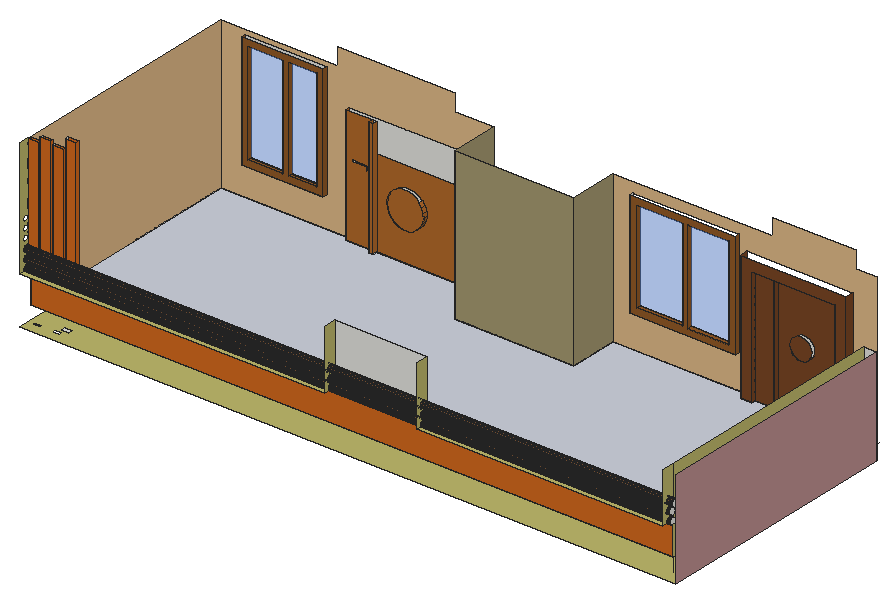
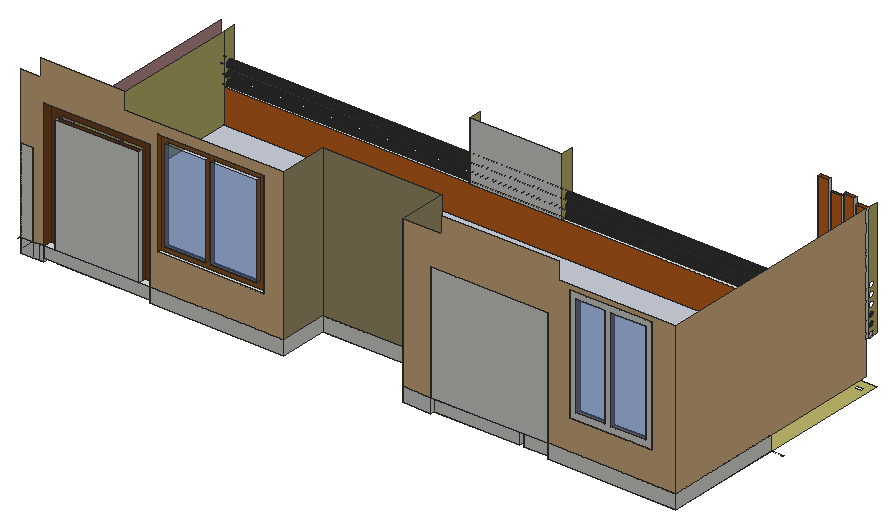
# SketchUp Ruby script. Lengths in inches.
U = 1.inch
M = Sketchup.active_model
def pt(a) = Geom::Point3d.new(a.map { |v| v * U })
def face(e, loops, mat)
  f = e.add_face(loops[0].map { |a| pt(a) })
  loops[1..].each { |l| e.add_face(l.map { |a| pt(a) }).erase! }
  f.material = f.back_material = mat if mat
  f
end
# faces: each face lists its corners as indices into pts; further lists are holes
def faces(e, pts, list, mat = nil) = list.each { |f| face(e, (f[0].is_a?(Array) ? f : [f]).map { |l| l.map { |i| pts[i] } }, mat) }
# xy, xz, yz: faces in a plane at the given z, y or x. An outline is a flat list of corners, or four numbers for a rectangle; further outlines are holes
def ring(l) = l.size == 4 ? [[l[0], l[1]], [l[2], l[1]], [l[2], l[3]], [l[0], l[3]]] : l.each_slice(2).to_a
def flat(e, list, mat, &to3) = list.each { |f| face(e, (f[0].is_a?(Array) ? f : [f]).map { |l| ring(l).map { |u, v| to3.(u, v) } }, mat) }
def xy(e, z, list, mat = nil) = flat(e, list, mat) { |x, y| [x, y, z] }
def xz(e, y, list, mat = nil) = flat(e, list, mat) { |x, z| [x, y, z] }
def yz(e, x, list, mat = nil) = flat(e, list, mat) { |y, z| [x, y, z] }
def lines(e, pts, list) = list.each { |a, b| e.add_line(pt(pts[a]), pt(pts[b])) }
# prism: a flat outline (further loops are holes) pulled along v
def prism(e, loops, v, mat = nil)
  f = face(e, loops, mat); d = Geom::Vector3d.new(v.map { |x| x * U })
  f.pushpull(f.normal.samedirection?(d) ? d.length : -d.length)
end
def box(e, o, s, mat = nil) = prism(e, [[o, [o[0] + s[0], o[1], o[2]], [o[0] + s[0], o[1] + s[1], o[2]], [o[0], o[1] + s[1], o[2]]]], [0, 0, s[2]], mat)
def at(x, y, z, deg = 0) = Geom::Transformation.translation(pt([x, y, z])) * Geom::Transformation.rotation(ORIGIN, Z_AXIS, deg.degrees)
def axes(o, x, y, z) = Geom::Transformation.new([*x, 0, *y, 0, *z, 0, *pt(o).to_a, 1])
def part(name) = M.definitions.add(name)
# library, detail: a bought-in or finely detailed component or shape, given as its bounding box
def library(name, o, s) = part(name).tap { |d| box(d.entities, o, s) }
def detail(e, o, s) = box(e.add_group.entities, o, s)
def put(e, d, t, mat = nil) = e.add_instance(d, t).tap { |i| i.material = mat if mat }
def group(e, t, mat = nil) = e.add_group.tap { |g| g.transformation = t; g.material = mat if mat }.entities
root = M.entities
M.materials.add("[0036_BurlyWood]").color = [222, 184, 135]
M.materials.add("[0041_Chocolate]").color = [210, 105, 30]
M.materials.add("[0057_DarkKhaki]").color = [189, 183, 107]
M.materials.add("[0119_RosyBrown]").color = [188, 143, 143]
M.materials.add("[Marble Carrara Floor Tile]").color = [204, 208, 219]
M.materials.add("[Sandstone]").color = [118, 81, 52]
M.materials.add("[Translucent Glass Blue]").color = [100, 149, 237]
M.materials["[Translucent Glass Blue]"].alpha = 0.5
M.materials.add("[Wood Bamboo]").color = [177, 105, 43]
M.materials.add("[Wood Floor Parquet]").color = [145, 89, 39]
M.materials.add("[Wood Lumber ButtJoined]").color = [164, 152, 112]
M.materials.add("[Wood Veneer 01]").color = [120, 70, 37]
xy(root,229.6875,[[[9,12,9,192.3,100.9,192.3,100.9,189.3,120.23,189.3,120.23,186.3,123.15,186.3,123.15,189.3,184.9,189.3,184.9,192.3,205.37,192.3,205.37,156.87,290.8125,156.87,290.8125,192.3,387.22,192.3,387.22,186.3,395.16,186.3,395.16,189.3,410.94,189.3,410.94,186.3,411.65,186.3,411.65,189.3,455.16,189.3,455.16,186.3,463.09,186.3,463.09,192.3,480,192.3,480,12],[12.36,18.25,17.86,21],[26.86,18.25,32.36,21]]],"[0057_DarkKhaki]")
xy(root,233.5625,[[33.61,18.25,39.11,21]])
xy(root,240,[[120.23,186.3,123.15,189.3],[387.22,186.3,395.16,192.3],[410.94,186.3,411.65,189.3],[455.16,186.3,463.09,192.3],[100.9,189.3,184.9,192.3],
  [395.16,189.3,455.16,192.3]])
xy(root,240,[[9,21,471,21,471,192.3,463.09,192.3,463.09,186.3,455.16,186.3,455.16,189.3,411.65,189.3,411.65,186.3,410.94,186.3,410.94,189.3,395.16,189.3,395.16,186.3,387.22,186.3,387.22,192.3,290.8125,192.3,290.8125,156.87,205.37,156.87,205.37,192.3,184.9,192.3,184.9,189.3,123.15,189.3,123.15,186.3,120.23,186.3,120.23,189.3,100.9,189.3,100.9,192.3,9,192.3]],"[Marble Carrara Floor Tile]")
xy(root,262.28,[[26.03,189.3,84.9,192.3]],"[Wood Floor Parquet]")
xy(root,264,[[9,15.41,227.54,18.4],[227.54,15.41,293.97,18.4],[293.97,15.41,471,18.4],[471,15.41,474.25,18.4],[9,18.4,227.54,18.4,227.54,21,43.6875,21,43.6875,18.8125,35.9375,18.8125,35.9375,21,34.6875,21,34.6875,18.8125,26.9375,18.8125,26.9375,21,25.5,21,25.5,18.8125,17.75,18.8125,17.75,21,16.75,21,16.75,18.8125,9,18.8125],
  [227.54,18.4,293.97,21],[293.97,18.4,471,21],[9,18.8125,16.75,21],[17.75,18.8125,25.5,21]])
xy(root,264,[[9,12,227.54,15.41],[293.97,12,471,15.41]],"[0057_DarkKhaki]")
xy(root,264.7,[[305.18,189.3,381.23,192.3]])
xy(root,266.72,[[30.47,189.3,55.47,192.3],[60.04,189.3,80.47,192.3]],"[Wood Floor Parquet]")
xy(root,269.51,[[309.99,189.3,343.2,192.3],[347.01,189.3,376.42,192.3]],"[Wood Floor Parquet]")
xz(root,18.8125,[[9,264,16.75,348],[17.75,264,25.5,351.875],[26.9375,264,34.6875,349.8125],[35.9375,264,43.6875,357.3125]],"[0041_Chocolate]")
xz(root,21,[[227.54,264,293.97,306.625]])
xz(root,21,[[9,240,9,264,26.9375,264,26.9375,349.8125,34.6875,349.8125,34.6875,264,35.9375,264,35.9375,357.3125,43.6875,357.3125,43.6875,264,471,264,471,240],[9,264,16.75,348],[17.75,264,25.5,351.875]],"[0041_Chocolate]")
xz(root,106.65,[[0,229.6875,9,229.8125]])
xz(root,156.87,[[205.37,229.6875,290.8125,240]])
xz(root,156.87,[[205.37,240,290.8125,348]],"[Wood Lumber ButtJoined]")
xz(root,186.3,[[120.23,229.6875,123.15,240],[387.22,229.6875,395.16,240],[410.94,229.6875,411.65,240],[455.16,229.6875,463.09,240]])
xz(root,186.3,[[120.23,240,123.15,324],[145.13,263.35,148.54,263.51,151.79,264.55,154.66,266.39,156.95,268.91,158.51,271.94,159.24,275.28,159.08,278.68,158.04,281.93,156.19,284.8,153.67,287.09,150.64,288.66,147.31,289.38,143.9,289.22,140.65,288.18,137.79,286.34,135.49,283.8125,133.93,280.78,133.2,277.45,133.37,274.04,134.4,270.8,136.25,267.93,138.77,265.63,141.8,264.07]],"[Wood Bamboo]")
xz(root,186.3,[[387.22,240,395.16,240,395.16,324,455.16,324,455.16,240,463.09,240,463.09,331.9375,387.22,331.9375],[410.94,240,411.65,324],[430.54,279.13,432.55,279.39,434.42,280.17,436.02,281.4,437.26,283,438.03,284.87,438.29,286.88,438.03,288.88,437.26,290.75,436.02,292.36,434.42,293.59,432.55,294.36,430.54,294.63,428.54,294.36,426.67,293.59,425.0625,292.36,423.83,290.75,423.06,288.88,422.79,286.88,423.06,284.87,423.83,283,425.0625,281.4,426.67,280.17,428.54,279.39]],"[Wood Veneer 01]")
xz(root,189.3,[[100.9,229.6875,120.23,240],[123.15,229.6875,184.9,240],[395.16,229.6875,410.94,240],[411.65,229.6875,455.16,240],[120.23,240,123.15,324],
  [410.94,240,411.65,324]])
xz(root,189.3,[[[100.9,240,120.23,324],[115.45,289,115.45,292.0625,105.14,292.0625,105.14,293.5,116.7,293.5,116.7,289]],[[123.15,240,184.9,303.1875],[145.13,263.35,141.8,264.07,138.77,265.63,136.25,267.93,134.4,270.8,133.37,274.04,133.2,277.45,133.93,280.78,135.49,283.8125,137.79,286.34,140.65,288.18,143.9,289.22,147.31,289.38,150.64,288.66,153.67,287.09,156.19,284.8,158.04,281.93,159.08,278.68,159.24,275.28,158.51,271.94,156.95,268.91,154.66,266.39,151.79,264.55,148.54,263.51]]],"[Wood Bamboo]")
xz(root,189.3,[[[26.03,262.28,84.9,344.59],[30.47,266.72,55.47,340.15],[60.04,266.72,80.47,340.15]],[[305.18,264.7,381.23,340.75],[309.99,269.51,343.2,335.94],[347.01,269.51,376.42,335.94]]],"[Wood Floor Parquet]")
xz(root,189.3,[[395.16,240,410.94,324],[[411.65,240,455.16,324],[430.54,279.13,428.54,279.39,426.67,280.17,425.0625,281.4,423.83,283,423.06,284.87,422.79,286.88,423.06,288.88,423.83,290.75,425.0625,292.36,426.67,293.59,428.54,294.36,430.54,294.63,432.55,294.36,434.42,293.59,436.02,292.36,437.26,290.75,438.03,288.88,438.29,286.88,438.03,284.87,437.26,283,436.02,281.4,434.42,280.17,432.55,279.39]]],"[Wood Veneer 01]")
xz(root,192.3,[[9,229.6875,100.9,240],[184.9,229.6875,205.37,240],[290.8125,229.6875,387.22,240],[463.09,229.6875,466.21,240],[466.21,229.6875,471,240],
  [471,229.6875,480,240],[387.22,232.0625,463.09,240],[100.9,240,184.9,324],[395.16,240,455.16,324],[471,240,480,300],
  [[26.03,262.28,84.9,344.59],[30.47,266.72,55.47,340.15],[60.04,266.72,80.47,340.15]]])
xz(root,192.3,[[[9,240,100.9,240,100.9,324,184.9,324,184.9,240,205.37,240,205.37,348,176.74,348,176.74,360,92.74,360,92.74,348,9,348],[26.03,262.28,84.9,344.59]],[[290.8125,240,387.22,240,387.22,331.9375,463.09,331.9375,463.09,240,471,240,471,300,480,300,480,348,465.34,348,465.34,360,405.34,360,405.34,348,290.8125,348],[305.18,264.7,381.23,340.75]]],"[0036_BurlyWood]")
xz(root,192.3,[[30.47,266.72,55.47,340.15],[60.04,266.72,80.47,340.15],[309.99,269.51,343.2,335.94],[347.01,269.51,376.42,335.94]],"[Translucent Glass Blue]")
yz(root,9,[[106.65,229.6875,192.3,240],[16.9,263.4,17.47,263.47,17.99,263.69,18.4,264,15.41,264,15.81,263.69,16.34,263.47],[15.41,264,15.35,264.04,15.01,264.49,14.79,265.02,14.71,265.59,14.79,266.15,15.01,266.68,15.35,267.13,15.81,267.48,16.34,267.7,16.9,267.77,17.47,267.7,17.99,267.48,18.45,267.13,18.8,266.68,18.8125,266.64,18.8125,264.53,18.8,264.49,18.45,264.04,18.4,264],[18.4,264,18.8125,264,18.8125,264.53,18.8,264.49,18.45,264.04],[18.8125,264,18.8125,264.53,19.01,265.02,19.09,265.59,19.01,266.15,18.8125,266.64,18.8125,348,21,348,21,264],
  [18.8125,264.53,18.8125,266.64,19.01,266.15,19.09,265.59,19.01,265.02]])
yz(root,9,[[21,240,192.3,348]],"[0036_BurlyWood]")
yz(root,9,[[[12,264,15.41,264,15.35,264.04,15.01,264.49,14.79,265.02,14.71,265.59,14.79,266.15,15.01,266.68,15.35,267.13,15.81,267.48,16.34,267.7,16.9,267.77,17.47,267.7,17.99,267.48,18.45,267.13,18.8,266.68,18.8125,266.64,18.8125,348,12,348],[16.59,295.27,16.03,295.35,15.5,295.57,15.04,295.91,14.7,296.37,14.48,296.9,14.4,297.46,14.48,298.03,14.7,298.56,15.04,299.01,15.5,299.36,16.03,299.57,16.59,299.65,17.16,299.57,17.69,299.36,18.14,299.01,18.49,298.56,18.7,298.03,18.78,297.46,18.7,296.9,18.49,296.37,18.14,295.91,17.69,295.57,17.16,295.35],[16.59,288.9,16.03,288.97,15.5,289.19,15.04,289.54,14.7,289.99,14.48,290.52,14.4,291.09,14.48,291.65,14.7,292.18,15.04,292.63,15.5,292.98,16.03,293.2,16.59,293.27,17.16,293.2,17.69,292.98,18.14,292.63,18.49,292.18,18.7,291.65,18.78,291.09,18.7,290.52,18.49,289.99,18.14,289.54,17.69,289.19,17.16,288.97],[16.59,282.52,16.03,282.6,15.5,282.82,15.04,283.16,14.7,283.62,14.48,284.15,14.4,284.71,14.48,285.28,14.7,285.81,15.04,286.26,15.5,286.61,16.03,286.82,16.59,286.9,17.16,286.82,17.69,286.61,18.14,286.26,18.49,285.81,18.7,285.28,18.78,284.71,18.7,284.15,18.49,283.62,18.14,283.16,17.69,282.82,17.16,282.6],[16.59,276.15,16.03,276.22,15.5,276.44,15.04,276.79,14.7,277.24,14.48,277.77,14.4,278.34,14.48,278.9,14.7,279.43,15.04,279.88,15.5,280.23,16.03,280.45,16.59,280.52,17.16,280.45,17.69,280.23,18.14,279.88,18.49,279.43,18.7,278.9,18.78,278.34,18.7,277.77,18.49,277.24,18.14,276.79,17.69,276.44,17.16,276.22],[16.59,269.77,16.03,269.85,15.5,270.07,15.04,270.41,14.7,270.87,14.48,271.4,14.4,271.96,14.48,272.53,14.7,273.06,15.04,273.51,15.5,273.86,16.03,274.07,16.59,274.15,17.16,274.07,17.69,273.86,18.14,273.51,18.49,273.06,18.7,272.53,18.78,271.96,18.7,271.4,18.49,270.87,18.14,270.41,17.69,270.07,17.16,269.85]]],"[0057_DarkKhaki]")
yz(root,16.75,[[18.8125,264,21,348]],"[0041_Chocolate]")
yz(root,17.75,[[18.8125,264,21,351.875]])
yz(root,25.5,[[18.8125,264,21,351.875]],"[0041_Chocolate]")
yz(root,26.03,[[189.3,262.28,192.3,344.59]],"[Wood Floor Parquet]")
yz(root,26.9375,[[18.8125,264,21,349.8125]])
yz(root,30.47,[[189.3,266.72,192.3,340.15]],"[Wood Floor Parquet]")
yz(root,34.6875,[[18.8125,264,21,349.8125]],"[0041_Chocolate]")
yz(root,35.9375,[[18.8125,264,21,357.3125]])
yz(root,43.6875,[[18.8125,264,21,357.3125]],"[0041_Chocolate]")
yz(root,55.47,[[189.3,266.72,192.3,340.15]],"[Wood Floor Parquet]")
yz(root,60.04,[[189.3,266.72,192.3,340.15]],"[Wood Floor Parquet]")
yz(root,80.47,[[189.3,266.72,192.3,340.15]],"[Wood Floor Parquet]")
yz(root,84.9,[[189.3,262.28,192.3,344.59]],"[Wood Floor Parquet]")
yz(root,100.9,[[189.3,229.6875,192.3,240]])
yz(root,100.9,[[189.3,240,192.3,324]],"[Wood Bamboo]")
yz(root,120.23,[[186.3,229.6875,189.3,240]])
yz(root,120.23,[[186.3,240,189.3,324]],"[Wood Bamboo]")
yz(root,123.15,[[186.3,229.6875,189.3,240]])
yz(root,123.15,[[186.3,240,189.3,324]],"[Wood Bamboo]")
yz(root,184.9,[[189.3,229.6875,192.3,240]])
yz(root,184.9,[[189.3,240,192.3,324]],"[Wood Bamboo]")
yz(root,205.37,[[156.87,229.6875,192.3,240]])
yz(root,205.37,[[156.87,240,192.3,348]],"[Wood Lumber ButtJoined]")
yz(root,227.54,[[12,264,21,306.625]],"[0057_DarkKhaki]")
yz(root,290.8125,[[156.87,229.6875,192.3,240]])
yz(root,290.8125,[[156.87,240,192.3,348]],"[Wood Lumber ButtJoined]")
yz(root,293.97,[[12,264,21,306.625]],"[0057_DarkKhaki]")
yz(root,305.18,[[189.3,264.7,192.3,340.75]])
yz(root,309.99,[[189.3,269.51,192.3,335.94]],"[Wood Floor Parquet]")
yz(root,343.2,[[189.3,269.51,192.3,335.94]],"[Wood Floor Parquet]")
yz(root,347.01,[[189.3,269.51,192.3,335.94]],"[Wood Floor Parquet]")
yz(root,376.42,[[189.3,269.51,192.3,335.94]],"[Wood Floor Parquet]")
yz(root,381.23,[[189.3,264.7,192.3,340.75]],"[Wood Floor Parquet]")
yz(root,387.22,[[186.3,229.6875,192.3,240]])
yz(root,387.22,[[186.3,240,192.3,331.9375]],"[Wood Veneer 01]")
yz(root,395.16,[[186.3,229.6875,189.3,240],[189.3,240,192.3,324]])
yz(root,395.16,[[186.3,240,189.3,324]],"[Wood Veneer 01]")
yz(root,410.94,[[186.3,229.6875,189.3,240]])
yz(root,410.94,[[186.3,240,189.3,324]],"[Wood Veneer 01]")
yz(root,411.65,[[186.3,229.6875,189.3,240]])
yz(root,411.65,[[186.3,240,189.3,324]],"[Wood Veneer 01]")
yz(root,455.16,[[186.3,229.6875,189.3,240],[189.3,240,192.3,324]])
yz(root,455.16,[[186.3,240,189.3,324]],"[Wood Veneer 01]")
yz(root,463.09,[[186.3,229.6875,192.3,240]])
yz(root,463.09,[[186.3,240,192.3,331.9375]],"[Wood Veneer 01]")
yz(root,471,[[21,240,192.3,300],[12,264,21,300]],"[0057_DarkKhaki]")
yz(root,473.8125,[[16.59,269.77,17.16,269.85,17.69,270.07,18.14,270.41,18.49,270.87,18.7,271.4,18.78,271.96,18.7,272.53,18.49,273.06,18.14,273.51,17.69,273.86,17.16,274.07,16.59,274.15,16.03,274.07,15.5,273.86,15.04,273.51,14.7,273.06,14.48,272.53,14.4,271.96,14.48,271.4,14.7,270.87,15.04,270.41,15.5,270.07,16.03,269.85]])
yz(root,474.25,[[15.41,264,18.4,264,18.45,264.04,18.8,264.49,19.01,265.02,19.09,265.59,19.01,266.15,18.8,266.68,18.45,267.13,17.99,267.48,17.47,267.7,16.9,267.77,16.34,267.7,15.81,267.48,15.35,267.13,15.01,266.68,14.79,266.15,14.71,265.59,14.79,265.02,15.01,264.49,15.35,264.04]])
yz(root,476.125,[[16.59,276.15,17.16,276.22,17.69,276.44,18.14,276.79,18.49,277.24,18.7,277.77,18.78,278.34,18.7,278.9,18.49,279.43,18.14,279.88,17.69,280.23,17.16,280.45,16.59,280.52,16.03,280.45,15.5,280.23,15.04,279.88,14.7,279.43,14.48,278.9,14.4,278.34,14.48,277.77,14.7,277.24,15.04,276.79,15.5,276.44,16.03,276.22]])
yz(root,480,[[12,229.6875,192.3,300]],"[0119_RosyBrown]")
p = [[141.8,189.3,264.07],[145.13,189.3,263.35],[145.13,186.3,263.35],[141.8,186.3,264.07],[148.54,189.3,263.51],[148.54,186.3,263.51],
  [151.79,189.3,264.55],[151.79,186.3,264.55],[9,15.01,264.49],[9,15.35,264.04],[474.25,15.35,264.04],[474.25,15.01,264.49],
  [9,15.41,264],[227.54,15.41,264],[293.97,15.41,264],[471,15.41,264],[474.25,15.41,264],[9,18.4,264],
  [9,18.45,264.04],[474.25,18.45,264.04],[474.25,18.4,264],[471,18.4,264],[293.97,18.4,264],[227.54,18.4,264],
  [9,18.8,264.49],[474.25,18.8,264.49],[138.77,189.3,265.63],[138.77,186.3,265.63],[9,14.79,265.02],[474.25,14.79,265.02],
  [9,18.8125,264.53],[9,19.01,265.02],[474.25,19.01,265.02],[154.66,189.3,266.39],[154.66,186.3,266.39],[9,14.71,265.59],
  [474.25,14.71,265.59],[9,19.09,265.59],[474.25,19.09,265.59],[9,14.79,266.15],[474.25,14.79,266.15],[9,19.01,266.15],
  [474.25,19.01,266.15],[136.25,189.3,267.93],[136.25,186.3,267.93],[9,15.01,266.68],[474.25,15.01,266.68],[9,18.8125,266.64],
  [9,18.8,266.68],[474.25,18.8,266.68],[156.95,189.3,268.91],[156.95,186.3,268.91],[9,15.35,267.13],[474.25,15.35,267.13],
  [9,18.45,267.13],[474.25,18.45,267.13],[9,15.81,267.48],[474.25,15.81,267.48],[9,17.99,267.48],[474.25,17.99,267.48],
  [9,16.34,267.7],[474.25,16.34,267.7],[9,17.47,267.7],[474.25,17.47,267.7],[9,16.9,267.77],[474.25,16.9,267.77],
  [134.4,189.3,270.8],[134.4,186.3,270.8],[158.51,189.3,271.94],[158.51,186.3,271.94],[9,15.5,270.07],[9,16.03,269.85],
  [473.8125,16.03,269.85],[473.8125,15.5,270.07],[9,16.59,269.77],[473.8125,16.59,269.77],[9,17.16,269.85],[473.8125,17.16,269.85],
  [9,17.69,270.07],[473.8125,17.69,270.07],[9,15.04,270.41],[473.8125,15.04,270.41],[9,18.14,270.41],[473.8125,18.14,270.41],
  [9,14.7,270.87],[473.8125,14.7,270.87],[9,18.49,270.87],[473.8125,18.49,270.87],[133.37,189.3,274.04],[133.37,186.3,274.04],
  [9,14.48,271.4],[473.8125,14.48,271.4],[9,18.7,271.4],[473.8125,18.7,271.4],[9,14.4,271.96],[473.8125,14.4,271.96],
  [9,18.78,271.96],[473.8125,18.78,271.96],[159.24,189.3,275.28],[159.24,186.3,275.28],[9,14.48,272.53],[473.8125,14.48,272.53],
  [9,18.7,272.53],[473.8125,18.7,272.53],[9,14.7,273.06],[473.8125,14.7,273.06],[9,18.49,273.06],[473.8125,18.49,273.06],
  [9,15.04,273.51],[473.8125,15.04,273.51],[9,18.14,273.51],[473.8125,18.14,273.51],[9,15.5,273.86],[473.8125,15.5,273.86],
  [9,17.69,273.86],[473.8125,17.69,273.86],[9,16.03,274.07],[473.8125,16.03,274.07],[9,17.16,274.07],[473.8125,17.16,274.07],
  [133.2,189.3,277.45],[133.2,186.3,277.45],[9,16.59,274.15],[473.8125,16.59,274.15],[159.08,189.3,278.68],[159.08,186.3,278.68],
  [9,16.03,276.22],[9,16.59,276.15],[476.125,16.59,276.15],[476.125,16.03,276.22],[9,17.16,276.22],[476.125,17.16,276.22],
  [9,15.5,276.44],[476.125,15.5,276.44],[9,17.69,276.44],[476.125,17.69,276.44],[9,15.04,276.79],[476.125,15.04,276.79],
  [9,18.14,276.79],[476.125,18.14,276.79],[9,14.7,277.24],[476.125,14.7,277.24],[9,18.49,277.24],[476.125,18.49,277.24],
  [9,14.48,277.77],[476.125,14.48,277.77],[9,18.7,277.77],[476.125,18.7,277.77],[133.93,189.3,280.78],[133.93,186.3,280.78],
  [9,14.4,278.34],[476.125,14.4,278.34],[9,18.78,278.34],[476.125,18.78,278.34],[9,14.48,278.9],[476.125,14.48,278.9],
  [9,18.7,278.9],[476.125,18.7,278.9],[158.04,189.3,281.93],[158.04,186.3,281.93],[9,14.7,279.43],[476.125,14.7,279.43],
  [9,18.49,279.43],[476.125,18.49,279.43],[428.54,189.3,279.39],[430.54,189.3,279.13],[430.54,186.3,279.13],[428.54,186.3,279.39],
  [432.55,189.3,279.39],[432.55,186.3,279.39],[9,15.04,279.88],[476.125,15.04,279.88],[9,18.14,279.88],[476.125,18.14,279.88],
  [426.67,189.3,280.17],[426.67,186.3,280.17],[434.42,189.3,280.17],[434.42,186.3,280.17],[9,15.5,280.23],[476.125,15.5,280.23],
  [9,17.69,280.23],[476.125,17.69,280.23],[9,16.03,280.45],[476.125,16.03,280.45],[9,17.16,280.45],[476.125,17.16,280.45],
  [425.0625,189.3,281.4],[425.0625,186.3,281.4],[436.02,189.3,281.4],[436.02,186.3,281.4],[9,16.59,280.52],[476.125,16.59,280.52],
  [135.49,189.3,283.8125],[135.49,186.3,283.8125],[423.83,189.3,283],[423.83,186.3,283],[437.26,189.3,283],[437.26,186.3,283],
  [156.19,189.3,284.8],[156.19,186.3,284.8],[471,316.59,240],[480,316.59,240],[480,195.03,240],[480,192.3,240],
  [471,195.03,240],[471,192.3,240],[471,201.23,240],[471,21,240],[471,21,229.6875]]
faces(root,p,[[0,1,2,3],[1,4,5,2],[4,6,7,5],[26,0,3,27],[6,33,34,7],[43,26,27,44],[33,50,51,34],[66,43,44,67],
  [50,68,69,51],[88,66,67,89],[68,98,99,69],[120,88,89,121],[98,124,125,99],[148,120,121,149],[124,158,159,125],[192,148,149,193],
  [158,198,199,159]],"[Wood Bamboo]")
faces(root,p,[[8,9,10,11],[9,12,13,14,15,16,10],[17,18,19,20,21,22,23],[18,24,25,19],[28,8,11,29],[30,31,32,25,24],[35,28,29,36],[31,37,38,32],
  [39,35,36,40],[37,41,42,38],[45,39,40,46],[47,48,49,42,41],[52,45,46,53],[48,54,55,49],[56,52,53,57],[54,58,59,55],
  [60,56,57,61],[58,62,63,59],[64,60,61,65],[62,64,65,63],[70,71,72,73],[71,74,75,72],[74,76,77,75],[76,78,79,77],
  [80,70,73,81],[78,82,83,79],[84,80,81,85],[82,86,87,83],[90,84,85,91],[86,92,93,87],[94,90,91,95],[92,96,97,93],
  [100,94,95,101],[96,102,103,97],[104,100,101,105],[102,106,107,103],[108,104,105,109],[106,110,111,107],[112,108,109,113],[110,114,115,111],
  [116,112,113,117],[114,118,119,115],[122,116,117,123],[118,122,123,119],[126,127,128,129],[127,130,131,128],[132,126,129,133],[130,134,135,131],
  [136,132,133,137],[134,138,139,135],[140,136,137,141],[138,142,143,139],[144,140,141,145],[142,146,147,143],[150,144,145,151],[146,152,153,147],
  [154,150,151,155],[152,156,157,153],[160,154,155,161],[156,162,163,157],[170,160,161,171],[162,172,173,163],[178,170,171,179],[172,180,181,173],
  [182,178,179,183],[180,184,185,181],[190,182,183,191],[184,190,191,185]],"[Sandstone]")
faces(root,p,[[164,165,166,167],[165,168,169,166],[174,164,167,175],[168,176,177,169],[186,174,175,187],[176,188,189,177],[194,186,187,195],[188,196,197,189]],"[Wood Veneer 01]")
lines(root,p,[[200,201],[202,203],[204,205],[206,204],[207,208]])
